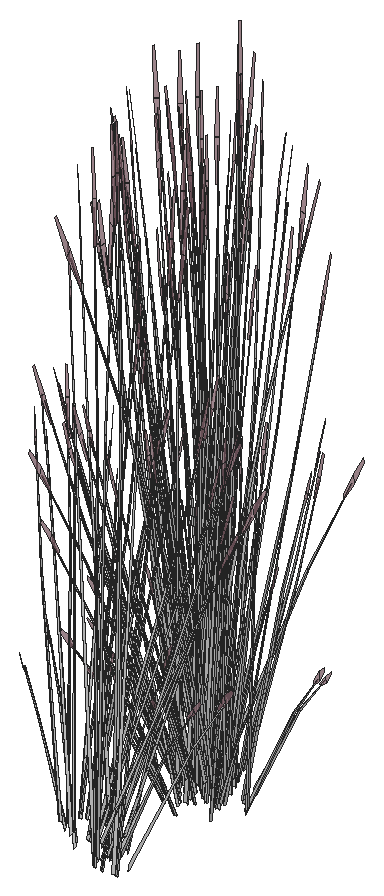
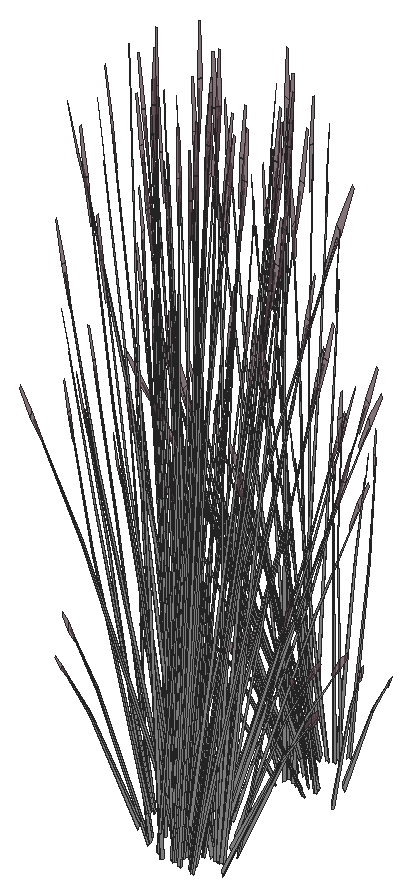
# SketchUp Ruby script. Lengths in inches.
U = 1.inch
M = Sketchup.active_model
def pt(a) = Geom::Point3d.new(a.map { |v| v * U })
def face(e, loops, mat)
  f = e.add_face(loops[0].map { |a| pt(a) })
  loops[1..].each { |l| e.add_face(l.map { |a| pt(a) }).erase! }
  f.material = f.back_material = mat if mat
  f
end
# faces: each face lists its corners as indices into pts; further lists are holes
def faces(e, pts, list, mat = nil) = list.each { |f| face(e, (f[0].is_a?(Array) ? f : [f]).map { |l| l.map { |i| pts[i] } }, mat) }
# xy, xz, yz: faces in a plane at the given z, y or x. An outline is a flat list of corners, or four numbers for a rectangle; further outlines are holes
def ring(l) = l.size == 4 ? [[l[0], l[1]], [l[2], l[1]], [l[2], l[3]], [l[0], l[3]]] : l.each_slice(2).to_a
def flat(e, list, mat, &to3) = list.each { |f| face(e, (f[0].is_a?(Array) ? f : [f]).map { |l| ring(l).map { |u, v| to3.(u, v) } }, mat) }
def xy(e, z, list, mat = nil) = flat(e, list, mat) { |x, y| [x, y, z] }
def xz(e, y, list, mat = nil) = flat(e, list, mat) { |x, z| [x, y, z] }
def yz(e, x, list, mat = nil) = flat(e, list, mat) { |y, z| [x, y, z] }
def lines(e, pts, list) = list.each { |a, b| e.add_line(pt(pts[a]), pt(pts[b])) }
# prism: a flat outline (further loops are holes) pulled along v
def prism(e, loops, v, mat = nil)
  f = face(e, loops, mat); d = Geom::Vector3d.new(v.map { |x| x * U })
  f.pushpull(f.normal.samedirection?(d) ? d.length : -d.length)
end
def box(e, o, s, mat = nil) = prism(e, [[o, [o[0] + s[0], o[1], o[2]], [o[0] + s[0], o[1] + s[1], o[2]], [o[0], o[1] + s[1], o[2]]]], [0, 0, s[2]], mat)
def at(x, y, z, deg = 0) = Geom::Transformation.translation(pt([x, y, z])) * Geom::Transformation.rotation(ORIGIN, Z_AXIS, deg.degrees)
def axes(o, x, y, z) = Geom::Transformation.new([*x, 0, *y, 0, *z, 0, *pt(o).to_a, 1])
def part(name) = M.definitions.add(name)
# library, detail: a bought-in or finely detailed component or shape, given as its bounding box
def library(name, o, s) = part(name).tap { |d| box(d.entities, o, s) }
def detail(e, o, s) = box(e.add_group.entities, o, s)
def put(e, d, t, mat = nil) = e.add_instance(d, t).tap { |i| i.material = mat if mat }
def group(e, t, mat = nil) = e.add_group.tap { |g| g.transformation = t; g.material = mat if mat }.entities
root = M.entities
M.materials.add("LightPink_Translucent").color = [144, 107, 117]
M.materials["LightPink_Translucent"].alpha = 0.75
M.materials.add("[_0053_Ivory_]").color = [200, 200, 200]
c1 = part("blade")
p = [[2.15,0.21,22],[0,0.17,0],[0.09,0.45,0],[2.18,0.31,22],[2.29,0.31,22],[0.38,0.45,0],
  [2.48,0.24,33],[2.49,0.24,33],[2.48,0.22,33]]
faces(c1.entities,p,[[0,1,2,3],[4,5,2,3],[6,3,4,7],[8,0,3,6]])
c2 = part("seeds")
p = [[0.3,-0.1,1.38],[-0.01,-0.03,1.59],[-0.01,-0.03,0.03],[0.14,-0.07,-0.07],[0.29,-0.03,3],[0.15,0.01,3.11]]
faces(c2.entities,p,[[0,1,2,3],[1,0,4,5]],"LightPink_Translucent")
c3 = part("blade with seeds")
put(c3.entities,c1,at(0,0,0))
put(c3.entities,c2,axes([2.4,0.25,30.99],[1.5799,-0.05474,1.17369],[-0.12525,1.92788,0.29478],[-0.07173,-0.02425,1.56792]))
put(root,c3,axes([640.09,126.82,129.42],[0.25312,-0.28501,1.1486],[0.09988,0.45119,0.84392],[-0.18292,0.08079,0.25299]),"[_0053_Ivory_]")
put(root,c3,axes([646.18,126.3,131.18],[0.34557,0.39372,-0.35414],[-0.39459,0.37271,0.4572],[0.20048,0.05671,0.87481]),"[_0053_Ivory_]")
put(root,c3,axes([646.35,125.2,128.68],[-0.42396,0.39235,-0.30978],[-0.42396,-0.39235,0.30978],[0,0.12637,1.38974]),"[_0053_Ivory_]")
put(root,c3,axes([644.52,125.24,129.32],[0.07077,0.71755,-0.29095],[-0.73712,0.04339,-0.50002],[-0.1298,0.09558,1.59708]),"[_0053_Ivory_]")
put(root,c3,axes([644.79,124.96,128.86],[-0.29468,0.56664,-0.44739],[-0.61229,-0.27271,0.21531],[0,0.13062,1.43643]),"[_0053_Ivory_]")
put(root,c3,axes([641.04,125.59,131.18],[-0.52868,0.08987,-0.35414],[-0.1396,-0.51376,0.4572],[-0.1515,0.13799,0.87481]),"[_0053_Ivory_]")
put(root,c3,axes([644.08,125.79,128.71],[-0.40909,0.47266,-0.62353],[-0.50819,-0.4286,-0.16365],[-0.16393,0.11791,1.37633]),"[_0053_Ivory_]")
put(root,c3,axes([644.81,126.59,128.98],[0.76036,0.2044,0.30756],[-0.19023,0.7306,-0.36492],[-0.12585,0.09144,1.64885]),"[_0053_Ivory_]")
put(root,c3,axes([644.75,127.08,128.67],[-0.56842,0.31443,-0.49651],[-0.33976,-0.56381,0],[-0.12946,0.07161,1.57504]),"[_0053_Ivory_]")
put(root,c3,axes([646.64,125.22,128.67],[0,0.62885,-0.49651],[-0.67951,0,0],[0,0.14322,1.57504]),"[_0053_Ivory_]")
put(root,c3,axes([644.94,125.29,130.53],[-0.2256,-0.10835,1.71376],[0.46687,-0.45453,0.13857],[0.29098,0.20505,0.73262]),"[_0053_Ivory_]")
put(root,c3,axes([645.78,126.52,129.42],[-0.34197,-0.18082,1.1486],[0.44156,-0.18372,0.84392],[0.1191,0.15563,0.25299]),"[_0053_Ivory_]")
put(root,c3,axes([641.96,125.09,130.53],[0.1517,-0.19322,1.71376],[0.38303,0.52154,0.13857],[-0.26271,0.23751,0.73262]),"[_0053_Ivory_]")
put(root,c3,axes([641.48,125.65,131.33],[0.15602,0.5742,-0.51099],[-0.59087,0.10045,-0.3958],[-0.16933,0.15423,0.97773]),"[_0053_Ivory_]")
put(root,c3,axes([645.27,126.98,129.03],[0.37973,0.63014,0],[-0.6353,0.35142,-0.51607],[-0.14469,0.08004,1.63711]),"[_0053_Ivory_]")
put(root,c3,axes([645.87,127.19,128.15],[0.04425,-0.09079,1.76342],[0.55709,-0.26738,-0.26939],[0.16889,0.13839,0.30037]),"[_0053_Ivory_]")
put(root,c3,axes([644.94,124.49,129.5],[-0.01659,-0.59209,1.41272],[0.75089,0.15348,0.59816],[-0.1776,0.32398,1.3335]),"[_0053_Ivory_]")
put(root,c3,axes([645.14,125.13,128.75],[0.2227,0.57576,-0.69212],[-0.64151,0.20736,-0.18165],[0.02462,0.19497,1.52773]),"[_0053_Ivory_]")
put(root,c3,axes([640.76,127.12,128.15],[0.08147,0.06283,1.76342],[0.13814,0.58211,-0.26939],[-0.18056,0.12413,0.30037]),"[_0053_Ivory_]")
put(root,c3,axes([645,126.77,131.33],[0.59932,-0.14948,-0.51099],[0.10484,0.56611,-0.3958],[0.16097,0.16223,0.97773]),"[_0053_Ivory_]")
put(root,c3,axes([645.83,127.34,129.32],[-0.38947,-0.01972,1.0506],[0.25721,-0.41888,0.58006],[0.15386,0.14882,0.8241]),"[_0053_Ivory_]")
put(root,c3,axes([641.84,125.5625,130.53],[0.11309,-0.21615,1.71376],[0.47441,0.44731,0.13857],[-0.21402,0.27879,0.73262]),"[_0053_Ivory_]")
put(root,c3,axes([644.56,126.33,129.24],[0.01072,-0.20846,1.43002],[0.51218,-0.23285,-0.30754],[0.15811,0.2495,0.61141]),"[_0053_Ivory_]")
put(root,c3,axes([641.97,126.78,131.18],[-0.41095,0.33109,-0.35414],[-0.38901,-0.37805,0.4572],[-0.05919,0.19208,0.87481]),"[_0053_Ivory_]")
put(root,c3,axes([642.24,128.07,129.42],[-0.01572,-0.37392,1.1486],[0.39276,0.26669,0.84392],[-0.07724,0.17822,0.25299]),"[_0053_Ivory_]")
put(root,c3,axes([643.27,127.17,128.15],[0.09829,-0.03422,1.76342],[0.59126,0.18834,-0.26939],[0.01729,0.21228,0.30037]),"[_0053_Ivory_]")
put(root,c3,axes([642.38,126.625,131.66],[0.43478,0.42253,-0.5672],[-0.45929,0.37004,-0.43934],[-0.06615,0.21468,1.08528]),"[_0053_Ivory_]")
put(root,c3,axes([641.91,127.26,129.48],[0.55175,-0.11136,0.06507],[0.12684,0.44864,-0.86304],[-0.03498,0.22711,0.7736]),"[_0053_Ivory_]")
put(root,c3,axes([643.67,127.03,131.33],[0.59704,0.15764,-0.51099],[-0.20464,0.54049,-0.3958],[0.05475,0.21761,0.97773]),"[_0053_Ivory_]")
put(root,c3,axes([644.01,125.92,130.53],[-0.13883,-0.2019,1.71376],[0.64153,-0.16998,0.13857],[0.14499,0.31697,0.73262]),"[_0053_Ivory_]")
put(root,c3,axes([642.49,136.88,130.53],[0.13883,0.2019,1.71376],[-0.64153,0.16998,0.13857],[-0.14499,-0.31697,0.73262]),"[_0053_Ivory_]")
put(root,c3,axes([643.4,127.36,131.18],[-0.1831,0.48359,-0.35414],[-0.53419,-0.14105,0.4572],[0.04898,0.1947,0.87481]),"[_0053_Ivory_]")
put(root,c3,axes([644.98,136.59,129.24],[-0.17264,0.12729,1.43002],[-0.51703,-0.22279,-0.30754],[0.09584,-0.27707,0.61141]),"[_0053_Ivory_]")
put(root,c3,axes([642.25,126.43,131.99],[-0.0158,0.58168,-0.7886],[-0.66548,-0.03907,0.09517],[-0.07023,0.24643,1.11556]),"[_0053_Ivory_]")
put(root,c3,axes([644.2,137.03,131.63],[-0.28988,-0.51132,-0.71045],[0.59671,-0.28496,0.08574],[-0.06778,-0.24706,1.00501]),"[_0053_Ivory_]")
put(root,c3,axes([642.3125,136.35,129.24],[-0.03678,0.20572,1.43002],[-0.53767,0.17221,-0.30754],[-0.12568,-0.26589,0.61141]),"[_0053_Ivory_]")
put(root,c3,axes([642.88,126.02,130.53],[-0.01487,-0.24136,1.71376],[0.64429,0.16012,0.13857],[-0.03985,0.34396,0.73262]),"[_0053_Ivory_]")
put(root,c3,axes([643.7,135.9,128.15],[-0.10187,0.02266,1.76342],[-0.56336,-0.25503,-0.26939],[0.00945,-0.21273,0.30037]),"[_0053_Ivory_]")
put(root,c3,axes([643.46,126.93,131.63],[0.28988,0.51132,-0.71045],[-0.59671,0.28496,0.08574],[0.06778,0.24706,1.00501]),"[_0053_Ivory_]")
put(root,c3,axes([645.4,137.53,131.63],[0.0158,-0.58168,-0.71045],[0.66548,0.03907,0.08574],[0.07023,-0.24643,1.00501]),"[_0053_Ivory_]")
put(root,c3,axes([641.78,127.73,129.24],[0.19166,-0.0992,1.43002],[0.4732,0.29912,-0.30754],[-0.14084,0.25882,0.61141]),"[_0053_Ivory_]")
put(root,c3,axes([644.25,136.6,131.18],[0.1831,-0.48359,-0.35414],[0.53419,0.14105,0.4572],[-0.04898,-0.1947,0.87481]),"[_0053_Ivory_]")
put(root,c3,axes([644.65,137.24,130.53],[-0.11309,0.21615,1.71376],[-0.47441,-0.44731,0.13857],[0.21402,-0.27879,0.73262]),"[_0053_Ivory_]")
put(root,c3,axes([643.98,136.93,131.33],[-0.59704,-0.15764,-0.51099],[0.20464,-0.54049,-0.3958],[-0.05475,-0.21761,0.97773]),"[_0053_Ivory_]")
put(root,c3,axes([644.35,135.57,129.42],[0.07791,0.3667,1.1486],[-0.43222,-0.2031,0.84392],[0.04651,-0.18776,0.25299]),"[_0053_Ivory_]")
put(root,c3,axes([645.27,137.34,131.33],[-0.43478,-0.42253,-0.51099],[0.45929,-0.37004,-0.3958],[0.06615,-0.21468,0.97773]),"[_0053_Ivory_]")
put(root,c3,axes([642.03,127.25,130.02],[0.01334,-0.32463,1.54345],[0.60018,0.17147,0.21329],[-0.052,0.34598,0.72882]),"[_0053_Ivory_]")
put(root,c3,axes([645.68,137.18,131.18],[0.41095,-0.33109,-0.35414],[0.38901,0.37805,0.4572],[0.05919,-0.19208,0.87481]),"[_0053_Ivory_]")
put(root,c3,axes([642.125,136.02,129.42],[0.31682,0.21887,1.1486],[-0.4614,0.13157,0.84392],[-0.09872,-0.16821,0.25299]),"[_0053_Ivory_]")
put(root,c3,axes([642.89,137.18,131.63],[-0.51789,-0.30395,-0.71045],[0.36805,-0.53263,0.08574],[-0.18764,-0.18149,1.00501]),"[_0053_Ivory_]")
put(root,c3,axes([642.71,136.77,131.18],[-0.0938,-0.50652,-0.35414],[0.53623,-0.13375,0.4572],[-0.14403,-0.14515,0.87481]),"[_0053_Ivory_]")
put(root,c3,axes([641.875,136.68,128.15],[-0.05883,0.08284,1.76342],[-0.59454,0.17861,-0.26939],[-0.14363,-0.16248,0.30037]),"[_0053_Ivory_]")
put(root,c3,axes([642.86,138.95,128.75],[-0.24943,-0.64486,-0.69835],[0.71849,-0.23224,-0.18329],[-0.02757,-0.21836,1.54149]),"[_0053_Ivory_]")
put(root,c3,axes([646.19,136.98,128.15],[-0.0909,-0.04954,1.76342],[-0.2335,-0.55347,-0.26939],[0.15752,-0.1502,0.30037]),"[_0053_Ivory_]")
put(root,c3,axes([642.65,137.19,131.33],[-0.59932,0.14948,-0.51099],[-0.10484,-0.56611,-0.3958],[-0.16097,-0.16223,0.97773]),"[_0053_Ivory_]")
put(root,c3,axes([646.1875,138.54,131.63],[0.31725,-0.49618,-0.71045],[0.55593,0.35263,0.08574],[0.18942,-0.17977,1.00501]),"[_0053_Ivory_]")
put(root,c3,axes([642.76,137.1,129.03],[-0.37973,-0.63014,0],[0.6353,-0.35142,-0.51607],[0.14469,-0.08004,1.63711]),"[_0053_Ivory_]")
put(root,c3,axes([646.17,138.31,131.33],[-0.15602,-0.5742,-0.51099],[0.59087,-0.10045,-0.3958],[0.16933,-0.15423,0.97773]),"[_0053_Ivory_]")
put(root,c3,axes([643.59,136.34,128.78],[-0.4197,0.36076,-0.03893],[-0.38456,-0.39511,-0.17649],[-0.02707,-0.11196,0.58215]),"[_0053_Ivory_]")
put(root,c3,axes([644.13,140.61,129.98],[0.52485,0.25358,1.51261],[-0.51417,0.54629,0.59816],[-0.23031,-0.32378,1.26806]),"[_0053_Ivory_]")
put(root,c3,axes([641.39,138.86,128.67],[0,-0.62885,-0.49651],[0.67951,0,0],[0,-0.14322,1.57504]),"[_0053_Ivory_]")
put(root,c3,axes([643.27,137,128.67],[0.56842,-0.31443,-0.49651],[0.33976,0.56381,0],[0.12946,-0.07161,1.57504]),"[_0053_Ivory_]")
put(root,c3,axes([646.65,138.09,129.24],[-0.21697,-0.01863,1.43002],[-0.22228,-0.49966,-0.30754],[0.26655,-0.14135,0.61141]),"[_0053_Ivory_]")
put(root,c3,axes([643.95,138.29,128.71],[0.40909,-0.47266,-0.62353],[0.50819,0.4286,-0.16365],[0.16393,-0.11791,1.37633]),"[_0053_Ivory_]")
put(root,c3,axes([646.9,137.17,129.42],[-0.2023,0.32011,1.1486],[-0.17388,-0.43009,0.84392],[0.16708,-0.10777,0.25299]),"[_0053_Ivory_]")
put(root,c3,axes([646.61,138.37,131.18],[0.52868,-0.08987,-0.35414],[0.1396,0.51376,0.4572],[0.1515,-0.13799,0.87481]),"[_0053_Ivory_]")
put(root,c3,axes([643.24,139.12,128.86],[0.29468,-0.56664,-0.44739],[0.61229,0.27271,0.21531],[0,-0.13062,1.43643]),"[_0053_Ivory_]")
put(root,c3,axes([641.47,137.66,131.18],[-0.34557,-0.39372,-0.35414],[0.39459,-0.37271,0.4572],[-0.20048,-0.05671,0.87481]),"[_0053_Ivory_]")
put(root,c3,axes([643.5,138.84,129.32],[-0.07077,-0.71755,-0.29095],[0.73712,-0.04339,-0.50002],[0.1298,-0.09558,1.59708]),"[_0053_Ivory_]")
put(root,c3,axes([641.68,138.875,128.68],[0.42396,-0.39235,-0.30978],[0.42396,0.39235,0.30978],[0,-0.12637,1.38974]),"[_0053_Ivory_]")
put(root,c3,axes([641.51,136.99,128.78],[-0.1752,0.51349,-0.03893],[-0.53924,-0.15795,-0.17649],[-0.08187,-0.08399,0.58215]),"[_0053_Ivory_]")
put(root,c3,axes([643.16,139.59,129.32],[-0.68399,-0.30005,-0.29095],[0.32934,-0.63331,-0.50002],[-0.0215,-0.15549,1.59708]),"[_0053_Ivory_]")
put(root,c3,axes([641.22,139.34,129.03],[-0.75945,0,0],[0,-0.70283,-0.51607],[0,-0.16007,1.63711]),"[_0053_Ivory_]")
put(root,c3,axes([643.41,137.25,128.68],[0.56663,0.1556,-0.30978],[-0.14267,0.54795,0.30978],[0.11423,-0.06319,1.38974]),"[_0053_Ivory_]")
put(root,c3,axes([641.8,139.15,128.98],[-0.56493,0.5287,0.30756],[-0.56528,-0.52313,-0.36492],[-0.01973,-0.15014,1.64885]),"[_0053_Ivory_]")
put(root,c3,axes([643.6,139.4,129.09],[0.68433,0.30479,0.24065],[-0.32934,0.63331,0.50002],[0,-0.14599,1.60543]),"[_0053_Ivory_]")
put(root,c3,axes([643.33,140.26,129.09],[0.16098,-0.74515,-0.23429],[0.76326,0.12989,0.51271],[-0.13337,-0.1029,1.5644]),"[_0053_Ivory_]")
put(root,c3,axes([640.64,138.61,129.42],[0.38775,-0.045,1.1486],[-0.24596,0.39648,0.84392],[-0.19161,-0.05948,0.25299]),"[_0053_Ivory_]")
put(root,c3,axes([643.38,138.97,129.37],[-0.65953,0.03882,0.44739],[-0.05964,-0.64439,-0.21531],[0.11807,-0.06531,1.43643]),"[_0053_Ivory_]")
put(root,c3,axes([641.68,139.45,129.13],[0,0.62885,0.49651],[-0.67951,0,0],[0,-0.14322,1.57504]),"[_0053_Ivory_]")
put(root,c3,axes([646.45,139.58,131.33],[0.16454,-0.57202,-0.51099],[0.56413,0.19607,-0.3958],[0.22713,-0.05245,0.97773]),"[_0053_Ivory_]")
put(root,c3,axes([645.55,137.26,129.03],[0.37973,-0.63014,0],[0.6353,0.35142,-0.51607],[0.14469,0.08004,1.63711]),"[_0053_Ivory_]")
put(root,c3,axes([643.28,139.95,128.86],[-0.36485,-0.52782,-0.44739],[0.55265,-0.37168,0.21531],[-0.11807,-0.06531,1.43643]),"[_0053_Ivory_]")
put(root,c3,axes([643.36,139.21,129.01],[0.26406,0.70318,0.45755],[-0.7545,0.24452,0.17955],[0.00922,-0.12921,1.58856]),"[_0053_Ivory_]")
put(root,c3,axes([647.05,139.75,128.64],[-0.39118,0.07547,1.41583],[-0.06226,-0.6007,0.08104],[0.27398,-0.09092,0.80566]),"[_0053_Ivory_]")
put(root,c3,axes([647.76,139.21,128.91],[-0.37654,-0.40212,-0.06488],[0.4124,-0.36845,-0.29416],[0.11685,-0.02594,0.97024]),"[_0053_Ivory_]")
put(root,c3,axes([643.22,139.76,129.37],[-0.29468,0.56664,0.44739],[-0.61229,-0.27271,-0.21531],[0,-0.13062,1.43643]),"[_0053_Ivory_]")
put(root,c3,axes([644.31,139.27,128.86],[0,-0.72763,0],[0.75945,0,0],[0,0,1.79456]),"[_0053_Ivory_]")
put(root,c3,axes([645.23,137.59,129.13],[-0.56842,-0.31443,0.49651],[0.33976,-0.56381,0],[0.12946,0.07161,1.57504]),"[_0053_Ivory_]")
put(root,c3,axes([646.34,139.79,131.63],[0.53369,-0.27773,-0.71045],[0.29743,0.5717,0.08574],[0.25786,-0.06494,1.00501]),"[_0053_Ivory_]")
put(root,c3,axes([642.95,140.15,128.71],[-0.63179,-0.1031,-0.62353],[0.13332,-0.63596,-0.16365],[-0.18854,-0.07706,1.37633]),"[_0053_Ivory_]")
put(root,c3,axes([643.95,138.81,129.01],[-0.50358,0.57069,0.45755],[-0.59827,-0.50377,0.17955],[0.1214,-0.05695,1.58856]),"[_0053_Ivory_]")
put(root,c3,axes([644.5,139.83,128.95],[-0.56493,-0.54126,-0.06131],[0.56528,-0.54159,0],[-0.01973,-0.0189,1.75571]),"[_0053_Ivory_]")
put(root,c3,axes([643.07,137.87,129.13],[-0.17545,0.62497,0.17642],[-0.64204,-0.17686,0.35086],[0.11091,-0.00304,1.60407]),"[_0053_Ivory_]")
put(root,c3,axes([642.81,138.37,128.25],[-0.59782,0.25177,1.28929],[-0.19028,-0.72239,0.50096],[0.36709,0.01202,1.46642]),"[_0053_Ivory_]")
put(root,c3,axes([644.41,138.5625,129.27],[0.11717,-0.56122,0.1448],[0.57245,0.09742,-0.41347],[0.10418,0.05763,1.26744]),"[_0053_Ivory_]")
put(root,c3,axes([643.42,139.9,129.01],[0.76764,0.13249,0.45755],[-0.15622,0.74829,0.17955],[-0.11218,-0.07226,1.58856]),"[_0053_Ivory_]")
put(root,c3,axes([647.48,139.35,128.15],[-0.03174,-0.09547,1.76342],[0.22015,-0.55846,-0.26939],[0.22208,-0.00803,0.30037]),"[_0053_Ivory_]")
put(root,c3,axes([640.92,139.26,128.15],[0.0154,0.09911,1.76342],[-0.31051,0.51756,-0.26939],[-0.22056,-0.02609,0.30037]),"[_0053_Ivory_]")
put(root,c3,axes([644.17,138.71,129.37],[-0.36485,-0.52782,0.44739],[0.55265,-0.37168,-0.21531],[0.11807,0.06531,1.43643]),"[_0053_Ivory_]")
put(root,c3,axes([642.28,141.125,128.68],[-0.14267,-0.54795,-0.30978],[0.56663,-0.1556,0.30978],[-0.11423,-0.06319,1.38974]),"[_0053_Ivory_]")
put(root,c3,axes([643.01,141.09,129.13],[0.65264,-0.16691,0.17642],[0.16115,0.62115,0.35086],[-0.05821,-0.0905,1.60407]),"[_0053_Ivory_]")
put(root,c3,axes([644.35,138.75,129.32],[0.61322,-0.4175,-0.29095],[0.40778,0.58992,-0.50002],[0.1513,0.05991,1.59708]),"[_0053_Ivory_]")
put(root,c3,axes([646.79,139.85,131.18],[0.50475,0.17543,-0.35414],[-0.14722,0.5118,0.4572],[0.20322,-0.04693,0.87481]),"[_0053_Ivory_]")
put(root,c3,axes([642.125,141.36,128.67],[-0.56842,-0.31443,-0.49651],[0.33976,-0.56381,0],[-0.12946,-0.07161,1.57504]),"[_0053_Ivory_]")
put(root,c3,axes([645.9,137.64,128.67],[0.56842,0.31443,-0.49651],[-0.33976,0.56381,0],[0.12946,0.07161,1.57504]),"[_0053_Ivory_]")
put(root,c3,axes([644.82,139.43,128.86],[0.67951,0,0],[0,0.65103,0],[0,0,1.78407]),"[_0053_Ivory_]")
put(root,c3,axes([643.67,140.25,129.32],[-0.61322,0.4175,-0.29095],[-0.40778,-0.58992,-0.50002],[-0.1513,-0.05991,1.59708]),"[_0053_Ivory_]")
put(root,c3,axes([645.01,137.9,129.13],[-0.65264,0.16691,0.17642],[-0.16115,-0.62115,0.35086],[0.05821,0.0905,1.60407]),"[_0053_Ivory_]")
put(root,c3,axes([645.42,139.21,130.53],[-0.25192,0.01424,1.71376],[0.16712,-0.61729,0.13857],[0.35901,0.03818,0.73262]),"[_0053_Ivory_]")
put(root,c3,axes([645.74,137.87,128.68],[0.14267,0.54795,-0.30978],[-0.56663,0.1556,0.30978],[0.11423,0.06319,1.38974]),"[_0053_Ivory_]")
put(root,c3,axes([644.6,139.1,129.03],[-0.76764,-0.13249,0.49198],[0.15622,-0.74829,0.19306],[0.11218,0.07226,1.70813]),"[_0053_Ivory_]")
put(root,c3,axes([643.99,140.95,128.86],[-0.19817,-0.54216,0],[0.56587,-0.18986,0],[0,0,1.54371]),"[_0053_Ivory_]")
put(root,c3,axes([643.61,140.43,129.27],[-0.11717,0.56122,0.1448],[-0.57245,-0.09742,-0.41347],[-0.10418,-0.05763,1.26744]),"[_0053_Ivory_]")
put(root,c3,axes([644.73,140.87,128.84],[0.63764,-0.21337,-0.19198],[0.22406,0.61462,0.00008],[0.07038,-0.02358,1.73897]),"[_0053_Ivory_]")
put(root,c3,axes([644.95,141.125,129.13],[0.17545,-0.62497,0.17642],[0.64204,0.17686,0.35086],[-0.11091,0.00304,1.60407]),"[_0053_Ivory_]")
put(root,c3,axes([644.81,139.71,128.87],[0.42396,0.40619,0],[-0.42396,0.40619,0],[0,0,1.69266]),"[_0053_Ivory_]")
put(root,c3,axes([645.95,139.53,129.13],[-0.47719,-0.45806,0.17642],[0.48088,-0.44429,0.35086],[-0.0527,0.09355,1.60407]),"[_0053_Ivory_]")
put(root,c3,axes([645.07,138.84,128.71],[0.63179,0.1031,-0.62353],[-0.13332,0.63596,-0.16365],[0.18854,0.07706,1.37633]),"[_0053_Ivory_]")
put(root,c3,axes([647.86,139.95,129.42],[-0.37526,0.10382,1.1486],[0.17664,-0.42906,0.84392],[0.19907,0.02936,0.25299]),"[_0053_Ivory_]")
put(root,c3,axes([643.85,141.19,128.85],[-0.61229,-0.28233,0],[0.29468,-0.58663,0],[0,0,1.62707]),"[_0053_Ivory_]")
put(root,c3,axes([644.36,140.4375,129.12],[-0.59306,-0.50614,-0.25192],[0.49904,-0.56836,0.5513],[-0.1597,0.05921,1.68216]),"[_0053_Ivory_]")
put(root,c3,axes([642.8,141.41,129.13],[0.56842,0.31443,0.49651],[-0.33976,0.56381,0],[-0.12946,-0.07161,1.57504]),"[_0053_Ivory_]")
put(root,c3,axes([644.8,139.23,129.37],[0.29468,-0.56664,0.44739],[0.61229,0.27271,-0.21531],[0,0.13062,1.43643]),"[_0053_Ivory_]")
put(root,c3,axes([644.6875,139.56,128.95],[0,0.72727,-0.05637],[-0.75945,0,0],[0,0.02286,1.79368]),"[_0053_Ivory_]")
